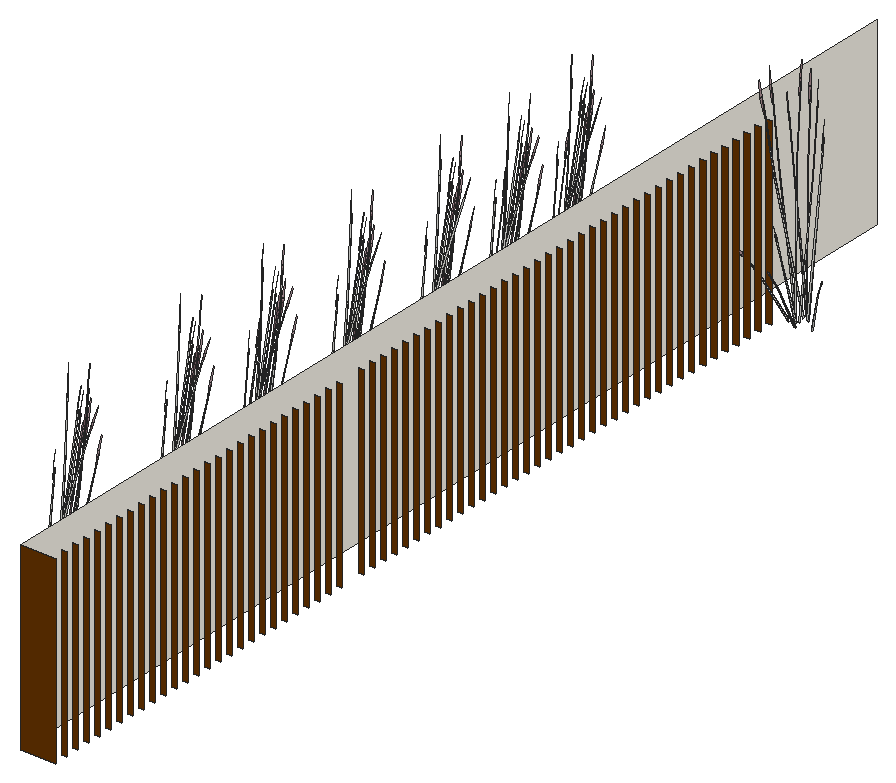
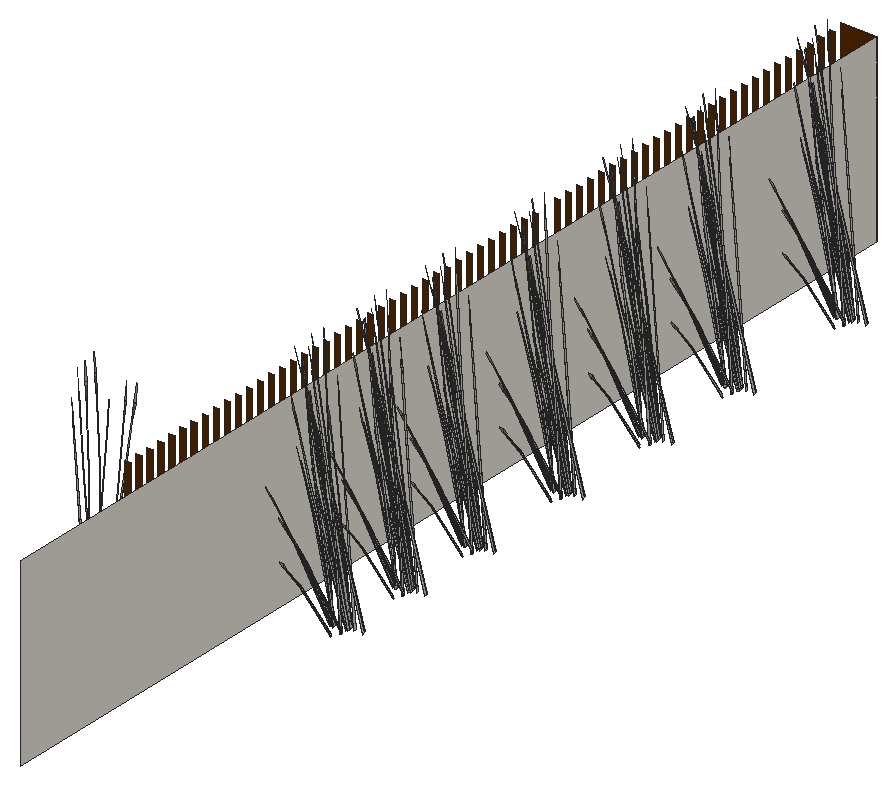
# SketchUp Ruby script. Lengths in inches.
U = 1.inch
M = Sketchup.active_model
def pt(a) = Geom::Point3d.new(a.map { |v| v * U })
def face(e, loops, mat)
  f = e.add_face(loops[0].map { |a| pt(a) })
  loops[1..].each { |l| e.add_face(l.map { |a| pt(a) }).erase! }
  f.material = f.back_material = mat if mat
  f
end
# faces: each face lists its corners as indices into pts; further lists are holes
def faces(e, pts, list, mat = nil) = list.each { |f| face(e, (f[0].is_a?(Array) ? f : [f]).map { |l| l.map { |i| pts[i] } }, mat) }
# xy, xz, yz: faces in a plane at the given z, y or x. An outline is a flat list of corners, or four numbers for a rectangle; further outlines are holes
def ring(l) = l.size == 4 ? [[l[0], l[1]], [l[2], l[1]], [l[2], l[3]], [l[0], l[3]]] : l.each_slice(2).to_a
def flat(e, list, mat, &to3) = list.each { |f| face(e, (f[0].is_a?(Array) ? f : [f]).map { |l| ring(l).map { |u, v| to3.(u, v) } }, mat) }
def xy(e, z, list, mat = nil) = flat(e, list, mat) { |x, y| [x, y, z] }
def xz(e, y, list, mat = nil) = flat(e, list, mat) { |x, z| [x, y, z] }
def yz(e, x, list, mat = nil) = flat(e, list, mat) { |y, z| [x, y, z] }
def lines(e, pts, list) = list.each { |a, b| e.add_line(pt(pts[a]), pt(pts[b])) }
# prism: a flat outline (further loops are holes) pulled along v
def prism(e, loops, v, mat = nil)
  f = face(e, loops, mat); d = Geom::Vector3d.new(v.map { |x| x * U })
  f.pushpull(f.normal.samedirection?(d) ? d.length : -d.length)
end
def box(e, o, s, mat = nil) = prism(e, [[o, [o[0] + s[0], o[1], o[2]], [o[0] + s[0], o[1] + s[1], o[2]], [o[0], o[1] + s[1], o[2]]]], [0, 0, s[2]], mat)
def at(x, y, z, deg = 0) = Geom::Transformation.translation(pt([x, y, z])) * Geom::Transformation.rotation(ORIGIN, Z_AXIS, deg.degrees)
def axes(o, x, y, z) = Geom::Transformation.new([*x, 0, *y, 0, *z, 0, *pt(o).to_a, 1])
def part(name) = M.definitions.add(name)
# library, detail: a bought-in or finely detailed component or shape, given as its bounding box
def library(name, o, s) = part(name).tap { |d| box(d.entities, o, s) }
def detail(e, o, s) = box(e.add_group.entities, o, s)
def put(e, d, t, mat = nil) = e.add_instance(d, t).tap { |i| i.material = mat if mat }
def group(e, t, mat = nil) = e.add_group.tap { |g| g.transformation = t; g.material = mat if mat }.entities
root = M.entities
M.materials.add("C01_Vanilla_Cream").color = [255, 251, 241]
M.materials.add("C08_Toffee_Ember").color = [102, 51, 0]
M.materials.add("LightPink_Translucent").color = [144, 107, 117]
M.materials["LightPink_Translucent"].alpha = 0.75
c1 = part("blade")
p = [[2.15,0.21,22],[0,0.17,0],[0.09,0.45,0],[2.18,0.31,22],[2.29,0.31,22],[0.38,0.45,0],
  [2.48,0.24,33],[2.49,0.24,33],[2.48,0.22,33]]
faces(c1.entities,p,[[0,1,2,3],[4,5,2,3],[6,3,4,7],[8,0,3,6]])
c2 = part("seeds")
p = [[0.3,-0.1,1.38],[-0.01,-0.03,1.59],[-0.01,-0.03,0.03],[0.14,-0.07,-0.07],[0.29,-0.03,3],[0.15,0.01,3.11]]
faces(c2.entities,p,[[0,1,2,3],[1,0,4,5]],"LightPink_Translucent")
c3 = part("blade with seeds")
put(c3.entities,c1,at(0,0,0))
put(c3.entities,c2,axes([2.4,0.25,30.99],[1.5799,-0.05474,1.17369],[-0.12525,1.92788,0.29478],[-0.07173,-0.02425,1.56792]))
xz(root,144,[[687.41,510,694.41,546]],"C08_Toffee_Ember")
xz(root,146.7,[[693.41,510,694.41,546]],"C08_Toffee_Ember")
xz(root,149.4,[[693.41,510,694.41,546]],"C08_Toffee_Ember")
xz(root,152.1,[[693.41,510,694.41,546]],"C08_Toffee_Ember")
xz(root,154.8,[[693.41,510,694.41,546]],"C08_Toffee_Ember")
xz(root,157.5,[[693.41,510,694.41,546]],"C08_Toffee_Ember")
xz(root,160.2,[[693.41,510,694.41,546]],"C08_Toffee_Ember")
xz(root,162.9,[[693.41,510,694.41,546]],"C08_Toffee_Ember")
xz(root,165.6,[[693.41,510,694.41,546]],"C08_Toffee_Ember")
xz(root,168.3,[[693.41,510,694.41,546]],"C08_Toffee_Ember")
xz(root,171,[[693.41,510,694.41,546]],"C08_Toffee_Ember")
xz(root,173.7,[[693.41,510,694.41,546]],"C08_Toffee_Ember")
xz(root,176.4,[[693.41,510,694.41,546]],"C08_Toffee_Ember")
xz(root,179.1,[[693.41,510,694.41,546]],"C08_Toffee_Ember")
xz(root,181.8,[[693.41,510,694.41,546]],"C08_Toffee_Ember")
xz(root,184.5,[[693.41,510,694.41,546]],"C08_Toffee_Ember")
xz(root,187.2,[[693.41,510,694.41,546]],"C08_Toffee_Ember")
xz(root,189.9,[[693.41,510,694.41,546]],"C08_Toffee_Ember")
xz(root,192.6,[[693.41,510,694.41,546]],"C08_Toffee_Ember")
xz(root,195.3,[[693.41,510,694.41,546]],"C08_Toffee_Ember")
xz(root,198,[[693.41,510,694.41,546]],"C08_Toffee_Ember")
xz(root,200.7,[[693.41,510,694.41,546]],"C08_Toffee_Ember")
xz(root,203.4,[[693.41,510,694.41,546]],"C08_Toffee_Ember")
xz(root,206.1,[[693.41,510,694.41,546]],"C08_Toffee_Ember")
xz(root,208.8,[[693.41,510,694.41,546]],"C08_Toffee_Ember")
xz(root,211.5,[[693.41,510,694.41,546]],"C08_Toffee_Ember")
xz(root,214.2,[[693.41,510,694.41,546]],"C08_Toffee_Ember")
xz(root,219.6,[[693.41,510,694.41,546]],"C08_Toffee_Ember")
xz(root,222.3,[[693.41,510,694.41,546]],"C08_Toffee_Ember")
xz(root,225,[[693.41,510,694.41,546]],"C08_Toffee_Ember")
xz(root,227.7,[[693.41,510,694.41,546]],"C08_Toffee_Ember")
xz(root,230.4,[[693.41,510,694.41,546]],"C08_Toffee_Ember")
xz(root,233.1,[[693.41,510,694.41,546]],"C08_Toffee_Ember")
xz(root,235.8,[[693.41,510,694.41,546]],"C08_Toffee_Ember")
xz(root,238.5,[[693.41,510,694.41,546]],"C08_Toffee_Ember")
xz(root,241.2,[[693.41,510,694.41,546]],"C08_Toffee_Ember")
xz(root,243.9,[[693.41,510,694.41,546]],"C08_Toffee_Ember")
xz(root,246.6,[[693.41,510,694.41,546]],"C08_Toffee_Ember")
xz(root,249.3,[[693.41,510,694.41,546]],"C08_Toffee_Ember")
xz(root,252,[[693.41,510,694.41,546]],"C08_Toffee_Ember")
xz(root,254.7,[[693.41,510,694.41,546]],"C08_Toffee_Ember")
xz(root,257.4,[[693.41,510,694.41,546]],"C08_Toffee_Ember")
xz(root,260.1,[[693.41,510,694.41,546]],"C08_Toffee_Ember")
xz(root,262.8,[[693.41,510,694.41,546]],"C08_Toffee_Ember")
xz(root,265.5,[[693.41,510,694.41,546]],"C08_Toffee_Ember")
xz(root,268.2,[[693.41,510,694.41,546]],"C08_Toffee_Ember")
xz(root,270.9,[[693.41,510,694.41,546]],"C08_Toffee_Ember")
xz(root,273.6,[[693.41,510,694.41,546]],"C08_Toffee_Ember")
xz(root,276.3,[[693.41,510,694.41,546]],"C08_Toffee_Ember")
xz(root,279,[[693.41,510,694.41,546]],"C08_Toffee_Ember")
xz(root,281.7,[[693.41,510,694.41,546]],"C08_Toffee_Ember")
xz(root,284.4,[[693.41,510,694.41,546]],"C08_Toffee_Ember")
xz(root,287.1,[[693.41,510,694.41,546]],"C08_Toffee_Ember")
xz(root,289.8,[[693.41,510,694.41,546]],"C08_Toffee_Ember")
xz(root,292.5,[[693.41,510,694.41,546]],"C08_Toffee_Ember")
xz(root,295.2,[[693.41,510,694.41,546]],"C08_Toffee_Ember")
xz(root,297.9,[[693.41,510,694.41,546]],"C08_Toffee_Ember")
xz(root,300.6,[[693.41,510,694.41,546]],"C08_Toffee_Ember")
xz(root,303.3,[[693.41,510,694.41,546]],"C08_Toffee_Ember")
xz(root,306,[[693.41,510,694.41,546]],"C08_Toffee_Ember")
xz(root,308.7,[[693.41,510,694.41,546]],"C08_Toffee_Ember")
xz(root,311.4,[[693.41,510,694.41,546]],"C08_Toffee_Ember")
xz(root,314.1,[[693.41,510,694.41,546]],"C08_Toffee_Ember")
xz(root,316.8,[[693.41,510,694.41,546]],"C08_Toffee_Ember")
xz(root,319.5,[[693.41,510,694.41,546]],"C08_Toffee_Ember")
yz(root,687.41,[[144,510,354,546]],"C01_Vanilla_Cream")
put(root,c3,axes([674.23,166.41,511.24],[-0.09738,-0.04498,1.46364],[-0.25012,-0.50252,-0.2236],[0.16873,-0.13637,0.24931]))
put(root,c3,axes([674.72,167.41,512.15],[-0.23242,-0.01691,1.18691],[-0.23811,-0.45367,-0.25526],[0.28553,-0.12834,0.50747]))
put(root,c3,axes([671.83,167.6,511.71],[0.43821,-0.42916,-0.51753],[0.54436,0.38915,-0.13583],[0.1756,-0.10706,1.14236]))
put(root,c3,axes([673.55,166.66,511.97],[0.40676,-0.57214,0],[0.68052,0.31907,-0.42834],[0.15499,0.07267,1.3588]))
put(root,c3,axes([675.15,168.92,511.65],[-0.41902,0.06852,1.17514],[-0.0667,-0.54541,0.06726],[0.29348,-0.08255,0.6687]))
put(root,c3,axes([675.92,168.4375,511.875],[-0.40335,-0.3651,-0.05385],[0.44175,-0.33453,-0.24415],[0.12517,-0.02355,0.8053]))
put(root,c3,axes([670.61,167.67,511.32],[-0.64037,0.22859,1.07011],[-0.20382,-0.65589,0.4158],[0.39323,0.01091,1.21713]))
put(root,c3,axes([675.61,168.5625,511.24],[-0.034,-0.08668,1.46364],[0.23582,-0.50706,-0.2236],[0.23788,-0.00729,0.24931]))
put(root,c3,axes([672.27,168.01,512.21],[0.65687,-0.37907,-0.24149],[0.43681,0.53562,-0.41502],[0.16207,0.0544,1.32557]))
put(root,c3,axes([673.92,167,511.67],[0.60889,0.28548,-0.4121],[-0.36394,0.51192,0],[0.13868,0.06502,1.30728]))
put(root,c3,axes([673.75,167.22,511.68],[0.15283,0.49751,-0.25712],[-0.60696,0.14127,0.25712],[0.12236,0.05737,1.15348]))
put(root,c3,axes([672.67,169.94,511.8125],[0.68303,-0.19373,-0.15934],[0.24001,0.55805,0.00007],[0.07539,-0.02141,1.44335]))
put(root,c3,axes([673.04,168.1,511.71],[0.67676,0.09361,-0.51753],[-0.14281,0.57742,-0.13583],[0.20196,0.06997,1.14236]))
put(root,c3,axes([672.68,168.28,511.83],[0.39083,0.47924,-0.37133],[-0.59199,0.33747,0.17871],[0.12647,0.0593,1.19224]))
put(root,c3,axes([675.27,169.73,512.15],[-0.15668,-0.14043,1.18691],[0.20386,-0.46454,-0.25526],[0.31701,0.06293,0.50747]))
put(root,c3,axes([674.9,168.84,511.97],[0.81352,0,0],[0,0.63814,-0.42834],[0,0.14534,1.3588]))
put(root,c3,axes([673.89,171.07,511.24],[0.0474,-0.08243,1.46364],[0.59674,-0.24277,-0.2236],[0.18092,0.12565,0.24931]))
put(root,c3,axes([672.49,170.28,512.15],[0.01148,-0.18927,1.18691],[0.54864,-0.21141,-0.25526],[0.16937,0.22654,0.50747]))
put(root,c3,axes([674.23,193.87,511.24],[-0.09738,-0.04498,1.46364],[-0.25012,-0.50252,-0.2236],[0.16873,-0.13637,0.24931]))
put(root,c3,axes([674.72,194.87,512.15],[-0.23242,-0.01691,1.18691],[-0.23811,-0.45367,-0.25526],[0.28553,-0.12834,0.50747]))
put(root,c3,axes([671.83,195.06,511.71],[0.43821,-0.42916,-0.51753],[0.54436,0.38915,-0.13583],[0.1756,-0.10706,1.14236]))
put(root,c3,axes([673.55,194.12,511.97],[0.40676,-0.57214,0],[0.68052,0.31907,-0.42834],[0.15499,0.07267,1.3588]))
put(root,c3,axes([675.15,196.38,511.65],[-0.41902,0.06852,1.17514],[-0.0667,-0.54541,0.06726],[0.29348,-0.08255,0.6687]))
put(root,c3,axes([675.92,195.9,511.875],[-0.40335,-0.3651,-0.05385],[0.44175,-0.33453,-0.24415],[0.12517,-0.02355,0.8053]))
put(root,c3,axes([670.61,195.13,511.32],[-0.64037,0.22859,1.07011],[-0.20382,-0.65589,0.4158],[0.39323,0.01091,1.21713]))
put(root,c3,axes([675.61,196.02,511.24],[-0.034,-0.08668,1.46364],[0.23582,-0.50706,-0.2236],[0.23788,-0.00729,0.24931]))
put(root,c3,axes([672.27,195.47,512.21],[0.65687,-0.37907,-0.24149],[0.43681,0.53562,-0.41502],[0.16207,0.0544,1.32557]))
put(root,c3,axes([673.92,194.46,511.67],[0.60889,0.28548,-0.4121],[-0.36394,0.51192,0],[0.13868,0.06502,1.30728]))
put(root,c3,axes([673.75,194.67,511.68],[0.15283,0.49751,-0.25712],[-0.60696,0.14127,0.25712],[0.12236,0.05737,1.15348]))
put(root,c3,axes([672.67,197.4,511.8125],[0.68303,-0.19373,-0.15934],[0.24001,0.55805,0.00007],[0.07539,-0.02141,1.44335]))
put(root,c3,axes([673.04,195.55,511.71],[0.67676,0.09361,-0.51753],[-0.14281,0.57742,-0.13583],[0.20196,0.06997,1.14236]))
put(root,c3,axes([672.68,195.74,511.83],[0.39083,0.47924,-0.37133],[-0.59199,0.33747,0.17871],[0.12647,0.0593,1.19224]))
put(root,c3,axes([675.27,197.1875,512.15],[-0.15668,-0.14043,1.18691],[0.20386,-0.46454,-0.25526],[0.31701,0.06293,0.50747]))
put(root,c3,axes([674.9,196.3,511.97],[0.81352,0,0],[0,0.63814,-0.42834],[0,0.14534,1.3588]))
put(root,c3,axes([673.89,198.52,511.24],[0.0474,-0.08243,1.46364],[0.59674,-0.24277,-0.2236],[0.18092,0.12565,0.24931]))
put(root,c3,axes([672.49,197.74,512.15],[0.01148,-0.18927,1.18691],[0.54864,-0.21141,-0.25526],[0.16937,0.22654,0.50747]))
put(root,c3,axes([674.23,214.16,511.24],[-0.09738,-0.04498,1.46364],[-0.25012,-0.50252,-0.2236],[0.16873,-0.13637,0.24931]))
put(root,c3,axes([674.72,215.16,512.15],[-0.23242,-0.01691,1.18691],[-0.23811,-0.45367,-0.25526],[0.28553,-0.12834,0.50747]))
put(root,c3,axes([671.83,215.35,511.71],[0.43821,-0.42916,-0.51753],[0.54436,0.38915,-0.13583],[0.1756,-0.10706,1.14236]))
put(root,c3,axes([673.55,214.41,511.97],[0.40676,-0.57214,0],[0.68052,0.31907,-0.42834],[0.15499,0.07267,1.3588]))
put(root,c3,axes([675.15,216.67,511.65],[-0.41902,0.06852,1.17514],[-0.0667,-0.54541,0.06726],[0.29348,-0.08255,0.6687]))
put(root,c3,axes([675.92,216.1875,511.875],[-0.40335,-0.3651,-0.05385],[0.44175,-0.33453,-0.24415],[0.12517,-0.02355,0.8053]))
put(root,c3,axes([670.61,215.42,511.32],[-0.64037,0.22859,1.07011],[-0.20382,-0.65589,0.4158],[0.39323,0.01091,1.21713]))
put(root,c3,axes([672.33,215.6,512.17],[0.12551,-0.50956,0.12018],[0.6132,0.08845,-0.34318],[0.1116,0.05232,1.05198]))
put(root,c3,axes([675.61,216.3125,511.24],[-0.034,-0.08668,1.46364],[0.23582,-0.50706,-0.2236],[0.23788,-0.00729,0.24931]))
put(root,c3,axes([672.27,215.76,512.21],[0.65687,-0.37907,-0.24149],[0.43681,0.53562,-0.41502],[0.16207,0.0544,1.32557]))
put(root,c3,axes([673.92,214.75,511.67],[0.60889,0.28548,-0.4121],[-0.36394,0.51192,0],[0.13868,0.06502,1.30728]))
put(root,c3,axes([673.75,214.97,511.68],[0.15283,0.49751,-0.25712],[-0.60696,0.14127,0.25712],[0.12236,0.05737,1.15348]))
put(root,c3,axes([672.67,217.69,511.8125],[0.68303,-0.19373,-0.15934],[0.24001,0.55805,0.00007],[0.07539,-0.02141,1.44335]))
put(root,c3,axes([673.04,215.85,511.71],[0.67676,0.09361,-0.51753],[-0.14281,0.57742,-0.13583],[0.20196,0.06997,1.14236]))
put(root,c3,axes([672.68,216.03,511.83],[0.39083,0.47924,-0.37133],[-0.59199,0.33747,0.17871],[0.12647,0.0593,1.19224]))
put(root,c3,axes([675.27,217.48,512.15],[-0.15668,-0.14043,1.18691],[0.20386,-0.46454,-0.25526],[0.31701,0.06293,0.50747]))
put(root,c3,axes([674.9,216.59,511.97],[0.81352,0,0],[0,0.63814,-0.42834],[0,0.14534,1.3588]))
put(root,c3,axes([673.89,218.82,511.24],[0.0474,-0.08243,1.46364],[0.59674,-0.24277,-0.2236],[0.18092,0.12565,0.24931]))
put(root,c3,axes([672.49,218.03,512.15],[0.01148,-0.18927,1.18691],[0.54864,-0.21141,-0.25526],[0.16937,0.22654,0.50747]))
put(root,c3,axes([674.23,235.86,511.24],[-0.09738,-0.04498,1.46364],[-0.25012,-0.50252,-0.2236],[0.16873,-0.13637,0.24931]))
put(root,c3,axes([674.72,236.86,512.15],[-0.23242,-0.01691,1.18691],[-0.23811,-0.45367,-0.25526],[0.28553,-0.12834,0.50747]))
put(root,c3,axes([671.83,237.04,511.71],[0.43821,-0.42916,-0.51753],[0.54436,0.38915,-0.13583],[0.1756,-0.10706,1.14236]))
put(root,c3,axes([673.55,236.11,511.97],[0.40676,-0.57214,0],[0.68052,0.31907,-0.42834],[0.15499,0.07267,1.3588]))
put(root,c3,axes([675.15,238.37,511.65],[-0.41902,0.06852,1.17514],[-0.0667,-0.54541,0.06726],[0.29348,-0.08255,0.6687]))
put(root,c3,axes([675.92,237.88,511.875],[-0.40335,-0.3651,-0.05385],[0.44175,-0.33453,-0.24415],[0.12517,-0.02355,0.8053]))
put(root,c3,axes([670.61,237.12,511.32],[-0.64037,0.22859,1.07011],[-0.20382,-0.65589,0.4158],[0.39323,0.01091,1.21713]))
put(root,c3,axes([675.61,238.01,511.24],[-0.034,-0.08668,1.46364],[0.23582,-0.50706,-0.2236],[0.23788,-0.00729,0.24931]))
put(root,c3,axes([672.27,237.46,512.21],[0.65687,-0.37907,-0.24149],[0.43681,0.53562,-0.41502],[0.16207,0.0544,1.32557]))
put(root,c3,axes([673.92,236.45,511.67],[0.60889,0.28548,-0.4121],[-0.36394,0.51192,0],[0.13868,0.06502,1.30728]))
put(root,c3,axes([673.75,236.66,511.68],[0.15283,0.49751,-0.25712],[-0.60696,0.14127,0.25712],[0.12236,0.05737,1.15348]))
put(root,c3,axes([672.67,239.39,511.8125],[0.68303,-0.19373,-0.15934],[0.24001,0.55805,0.00007],[0.07539,-0.02141,1.44335]))
put(root,c3,axes([673.04,237.54,511.71],[0.67676,0.09361,-0.51753],[-0.14281,0.57742,-0.13583],[0.20196,0.06997,1.14236]))
put(root,c3,axes([672.68,237.73,511.83],[0.39083,0.47924,-0.37133],[-0.59199,0.33747,0.17871],[0.12647,0.0593,1.19224]))
put(root,c3,axes([675.27,239.18,512.15],[-0.15668,-0.14043,1.18691],[0.20386,-0.46454,-0.25526],[0.31701,0.06293,0.50747]))
put(root,c3,axes([674.9,238.29,511.97],[0.81352,0,0],[0,0.63814,-0.42834],[0,0.14534,1.3588]))
put(root,c3,axes([673.89,240.51,511.24],[0.0474,-0.08243,1.46364],[0.59674,-0.24277,-0.2236],[0.18092,0.12565,0.24931]))
put(root,c3,axes([672.49,239.73,512.15],[0.01148,-0.18927,1.18691],[0.54864,-0.21141,-0.25526],[0.16937,0.22654,0.50747]))
put(root,c3,axes([674.23,257.7,511.24],[-0.09738,-0.04498,1.46364],[-0.25012,-0.50252,-0.2236],[0.16873,-0.13637,0.24931]))
put(root,c3,axes([674.72,258.71,512.15],[-0.23242,-0.01691,1.18691],[-0.23811,-0.45367,-0.25526],[0.28553,-0.12834,0.50747]))
put(root,c3,axes([671.83,258.89,511.71],[0.43821,-0.42916,-0.51753],[0.54436,0.38915,-0.13583],[0.1756,-0.10706,1.14236]))
put(root,c3,axes([673.55,257.95,511.97],[0.40676,-0.57214,0],[0.68052,0.31907,-0.42834],[0.15499,0.07267,1.3588]))
put(root,c3,axes([675.15,260.21,511.65],[-0.41902,0.06852,1.17514],[-0.0667,-0.54541,0.06726],[0.29348,-0.08255,0.6687]))
put(root,c3,axes([675.92,259.73,511.875],[-0.40335,-0.3651,-0.05385],[0.44175,-0.33453,-0.24415],[0.12517,-0.02355,0.8053]))
put(root,c3,axes([670.61,258.97,511.32],[-0.64037,0.22859,1.07011],[-0.20382,-0.65589,0.4158],[0.39323,0.01091,1.21713]))
put(root,c3,axes([675.61,259.86,511.24],[-0.034,-0.08668,1.46364],[0.23582,-0.50706,-0.2236],[0.23788,-0.00729,0.24931]))
put(root,c3,axes([672.27,259.3,512.21],[0.65687,-0.37907,-0.24149],[0.43681,0.53562,-0.41502],[0.16207,0.0544,1.32557]))
put(root,c3,axes([673.92,258.3,511.67],[0.60889,0.28548,-0.4121],[-0.36394,0.51192,0],[0.13868,0.06502,1.30728]))
put(root,c3,axes([673.75,258.51,511.68],[0.15283,0.49751,-0.25712],[-0.60696,0.14127,0.25712],[0.12236,0.05737,1.15348]))
put(root,c3,axes([672.67,261.23,511.8125],[0.68303,-0.19373,-0.15934],[0.24001,0.55805,0.00007],[0.07539,-0.02141,1.44335]))
put(root,c3,axes([673.04,259.39,511.71],[0.67676,0.09361,-0.51753],[-0.14281,0.57742,-0.13583],[0.20196,0.06997,1.14236]))
put(root,c3,axes([672.68,259.57,511.83],[0.39083,0.47924,-0.37133],[-0.59199,0.33747,0.17871],[0.12647,0.0593,1.19224]))
put(root,c3,axes([675.27,261.02,512.15],[-0.15668,-0.14043,1.18691],[0.20386,-0.46454,-0.25526],[0.31701,0.06293,0.50747]))
put(root,c3,axes([674.9,260.13,511.97],[0.81352,0,0],[0,0.63814,-0.42834],[0,0.14534,1.3588]))
put(root,c3,axes([673.89,262.36,511.24],[0.0474,-0.08243,1.46364],[0.59674,-0.24277,-0.2236],[0.18092,0.12565,0.24931]))
put(root,c3,axes([672.49,261.57,512.15],[0.01148,-0.18927,1.18691],[0.54864,-0.21141,-0.25526],[0.16937,0.22654,0.50747]))
put(root,c3,axes([674.23,274.5625,511.24],[-0.09738,-0.04498,1.46364],[-0.25012,-0.50252,-0.2236],[0.16873,-0.13637,0.24931]))
put(root,c3,axes([674.72,275.56,512.15],[-0.23242,-0.01691,1.18691],[-0.23811,-0.45367,-0.25526],[0.28553,-0.12834,0.50747]))
put(root,c3,axes([671.83,275.75,511.71],[0.43821,-0.42916,-0.51753],[0.54436,0.38915,-0.13583],[0.1756,-0.10706,1.14236]))
put(root,c3,axes([673.55,274.8125,511.97],[0.40676,-0.57214,0],[0.68052,0.31907,-0.42834],[0.15499,0.07267,1.3588]))
put(root,c3,axes([675.15,277.07,511.65],[-0.41902,0.06852,1.17514],[-0.0667,-0.54541,0.06726],[0.29348,-0.08255,0.6687]))
put(root,c3,axes([675.92,276.59,511.875],[-0.40335,-0.3651,-0.05385],[0.44175,-0.33453,-0.24415],[0.12517,-0.02355,0.8053]))
put(root,c3,axes([670.61,275.83,511.32],[-0.64037,0.22859,1.07011],[-0.20382,-0.65589,0.4158],[0.39323,0.01091,1.21713]))
put(root,c3,axes([672.33,276,512.17],[0.12551,-0.50956,0.12018],[0.6132,0.08845,-0.34318],[0.1116,0.05232,1.05198]))
put(root,c3,axes([675.61,276.72,511.24],[-0.034,-0.08668,1.46364],[0.23582,-0.50706,-0.2236],[0.23788,-0.00729,0.24931]))
put(root,c3,axes([672.27,276.16,512.21],[0.65687,-0.37907,-0.24149],[0.43681,0.53562,-0.41502],[0.16207,0.0544,1.32557]))
put(root,c3,axes([673.92,275.16,511.67],[0.60889,0.28548,-0.4121],[-0.36394,0.51192,0],[0.13868,0.06502,1.30728]))
put(root,c3,axes([673.75,275.37,511.68],[0.15283,0.49751,-0.25712],[-0.60696,0.14127,0.25712],[0.12236,0.05737,1.15348]))
put(root,c3,axes([672.67,278.09,511.8125],[0.68303,-0.19373,-0.15934],[0.24001,0.55805,0.00007],[0.07539,-0.02141,1.44335]))
put(root,c3,axes([673.04,276.25,511.71],[0.67676,0.09361,-0.51753],[-0.14281,0.57742,-0.13583],[0.20196,0.06997,1.14236]))
put(root,c3,axes([672.68,276.43,511.83],[0.39083,0.47924,-0.37133],[-0.59199,0.33747,0.17871],[0.12647,0.0593,1.19224]))
put(root,c3,axes([675.27,277.88,512.15],[-0.15668,-0.14043,1.18691],[0.20386,-0.46454,-0.25526],[0.31701,0.06293,0.50747]))
put(root,c3,axes([674.9,276.99,511.97],[0.81352,0,0],[0,0.63814,-0.42834],[0,0.14534,1.3588]))
put(root,c3,axes([673.89,279.22,511.24],[0.0474,-0.08243,1.46364],[0.59674,-0.24277,-0.2236],[0.18092,0.12565,0.24931]))
put(root,c3,axes([672.49,278.43,512.15],[0.01148,-0.18927,1.18691],[0.54864,-0.21141,-0.25526],[0.16937,0.22654,0.50747]))
put(root,c3,axes([674.23,289.9,511.24],[-0.09738,-0.04498,1.46364],[-0.25012,-0.50252,-0.2236],[0.16873,-0.13637,0.24931]))
put(root,c3,axes([674.72,290.9,512.15],[-0.23242,-0.01691,1.18691],[-0.23811,-0.45367,-0.25526],[0.28553,-0.12834,0.50747]))
put(root,c3,axes([671.83,291.08,511.71],[0.43821,-0.42916,-0.51753],[0.54436,0.38915,-0.13583],[0.1756,-0.10706,1.14236]))
put(root,c3,axes([673.55,290.15,511.97],[0.40676,-0.57214,0],[0.68052,0.31907,-0.42834],[0.15499,0.07267,1.3588]))
put(root,c3,axes([675.15,292.41,511.65],[-0.41902,0.06852,1.17514],[-0.0667,-0.54541,0.06726],[0.29348,-0.08255,0.6687]))
put(root,c3,axes([675.92,291.92,511.875],[-0.40335,-0.3651,-0.05385],[0.44175,-0.33453,-0.24415],[0.12517,-0.02355,0.8053]))
put(root,c3,axes([670.61,291.16,511.32],[-0.64037,0.22859,1.07011],[-0.20382,-0.65589,0.4158],[0.39323,0.01091,1.21713]))
put(root,c3,axes([672.33,291.33,512.17],[0.12551,-0.50956,0.12018],[0.6132,0.08845,-0.34318],[0.1116,0.05232,1.05198]))
put(root,c3,axes([675.61,292.05,511.24],[-0.034,-0.08668,1.46364],[0.23582,-0.50706,-0.2236],[0.23788,-0.00729,0.24931]))
put(root,c3,axes([672.27,291.5,512.21],[0.65687,-0.37907,-0.24149],[0.43681,0.53562,-0.41502],[0.16207,0.0544,1.32557]))
put(root,c3,axes([673.92,290.49,511.67],[0.60889,0.28548,-0.4121],[-0.36394,0.51192,0],[0.13868,0.06502,1.30728]))
put(root,c3,axes([673.75,290.7,511.68],[0.15283,0.49751,-0.25712],[-0.60696,0.14127,0.25712],[0.12236,0.05737,1.15348]))
put(root,c3,axes([672.67,293.43,511.8125],[0.68303,-0.19373,-0.15934],[0.24001,0.55805,0.00007],[0.07539,-0.02141,1.44335]))
put(root,c3,axes([673.04,291.58,511.71],[0.67676,0.09361,-0.51753],[-0.14281,0.57742,-0.13583],[0.20196,0.06997,1.14236]))
put(root,c3,axes([672.68,291.77,511.83],[0.39083,0.47924,-0.37133],[-0.59199,0.33747,0.17871],[0.12647,0.0593,1.19224]))
put(root,c3,axes([675.27,293.22,512.15],[-0.15668,-0.14043,1.18691],[0.20386,-0.46454,-0.25526],[0.31701,0.06293,0.50747]))
put(root,c3,axes([674.9,292.32,511.97],[0.81352,0,0],[0,0.63814,-0.42834],[0,0.14534,1.3588]))
put(root,c3,axes([673.89,294.55,511.24],[0.0474,-0.08243,1.46364],[0.59674,-0.24277,-0.2236],[0.18092,0.12565,0.24931]))
put(root,c3,axes([672.49,293.77,512.15],[0.01148,-0.18927,1.18691],[0.54864,-0.21141,-0.25526],[0.16937,0.22654,0.50747]))
put(root,c3,axes([699.17,319.6,511.24],[-0.10912,0.02057,1.46364],[-0.60346,-0.23156,-0.2236],[0.01013,-0.19315,0.24931]))
put(root,c3,axes([697.22,320.31,511.24],[-0.06302,0.07522,1.46364],[-0.63686,0.16217,-0.2236],[-0.15385,-0.14752,0.24931]))
put(root,c3,axes([698.27,322.375,511.74],[-0.26718,-0.5855,-0.57963],[0.76964,-0.21087,-0.15213],[-0.02953,-0.19827,1.27944]))
put(root,c3,axes([701.84,320.59,511.24],[-0.09738,-0.04498,1.46364],[-0.25012,-0.50252,-0.2236],[0.16873,-0.13637,0.24931]))
put(root,c3,axes([698.16,320.69,511.97],[-0.40676,-0.57214,0],[0.68052,-0.31907,-0.42834],[0.15499,-0.07267,1.3588]))
put(root,c3,axes([699.06,320,511.77],[-0.44958,0.32756,-0.03231],[-0.41194,-0.35875,-0.14649],[-0.029,-0.10165,0.48318]))
put(root,c3,axes([696.69,322.29,511.67],[0,-0.57097,-0.4121],[0.72788,0,0],[0,-0.13004,1.30728]))
put(root,c3,axes([698.72,320.6,511.67],[0.60889,-0.28548,-0.4121],[0.36394,0.51192,0],[0.13868,-0.06502,1.30728]))
put(root,c3,axes([699.4375,321.78,511.71],[0.43821,-0.42916,-0.51753],[0.54436,0.38915,-0.13583],[0.1756,-0.10706,1.14236]))
put(root,c3,axes([698.67,322.53,511.83],[0.31565,-0.51449,-0.37133],[0.65588,0.24761,0.17871],[0,-0.1186,1.19224]))
put(root,c3,axes([698.96,322.27,512.21],[-0.07581,-0.65151,-0.24149],[0.7896,-0.03939,-0.41502],[0.13904,-0.08678,1.32557]))
